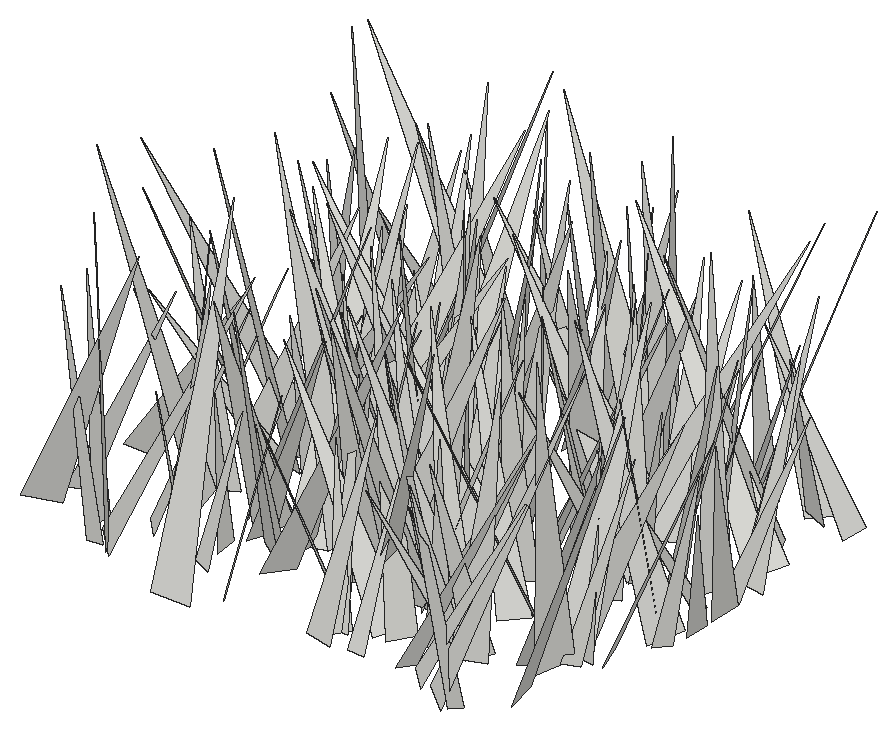
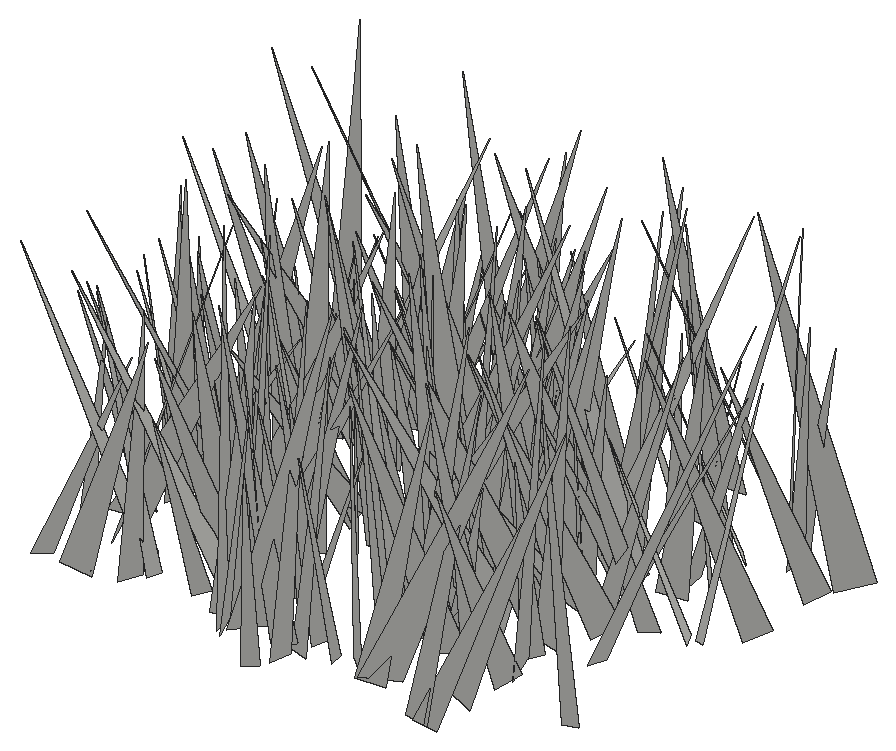
# SketchUp Ruby script. Lengths in inches.
U = 1.inch
M = Sketchup.active_model
def pt(a) = Geom::Point3d.new(a.map { |v| v * U })
def face(e, loops, mat)
  f = e.add_face(loops[0].map { |a| pt(a) })
  loops[1..].each { |l| e.add_face(l.map { |a| pt(a) }).erase! }
  f.material = f.back_material = mat if mat
  f
end
# faces: each face lists its corners as indices into pts; further lists are holes
def faces(e, pts, list, mat = nil) = list.each { |f| face(e, (f[0].is_a?(Array) ? f : [f]).map { |l| l.map { |i| pts[i] } }, mat) }
# xy, xz, yz: faces in a plane at the given z, y or x. An outline is a flat list of corners, or four numbers for a rectangle; further outlines are holes
def ring(l) = l.size == 4 ? [[l[0], l[1]], [l[2], l[1]], [l[2], l[3]], [l[0], l[3]]] : l.each_slice(2).to_a
def flat(e, list, mat, &to3) = list.each { |f| face(e, (f[0].is_a?(Array) ? f : [f]).map { |l| ring(l).map { |u, v| to3.(u, v) } }, mat) }
def xy(e, z, list, mat = nil) = flat(e, list, mat) { |x, y| [x, y, z] }
def xz(e, y, list, mat = nil) = flat(e, list, mat) { |x, z| [x, y, z] }
def yz(e, x, list, mat = nil) = flat(e, list, mat) { |y, z| [x, y, z] }
def lines(e, pts, list) = list.each { |a, b| e.add_line(pt(pts[a]), pt(pts[b])) }
# prism: a flat outline (further loops are holes) pulled along v
def prism(e, loops, v, mat = nil)
  f = face(e, loops, mat); d = Geom::Vector3d.new(v.map { |x| x * U })
  f.pushpull(f.normal.samedirection?(d) ? d.length : -d.length)
end
def box(e, o, s, mat = nil) = prism(e, [[o, [o[0] + s[0], o[1], o[2]], [o[0] + s[0], o[1] + s[1], o[2]], [o[0], o[1] + s[1], o[2]]]], [0, 0, s[2]], mat)
def at(x, y, z, deg = 0) = Geom::Transformation.translation(pt([x, y, z])) * Geom::Transformation.rotation(ORIGIN, Z_AXIS, deg.degrees)
def axes(o, x, y, z) = Geom::Transformation.new([*x, 0, *y, 0, *z, 0, *pt(o).to_a, 1])
def part(name) = M.definitions.add(name)
# library, detail: a bought-in or finely detailed component or shape, given as its bounding box
def library(name, o, s) = part(name).tap { |d| box(d.entities, o, s) }
def detail(e, o, s) = box(e.add_group.entities, o, s)
def put(e, d, t, mat = nil) = e.add_instance(d, t).tap { |i| i.material = mat if mat }
def group(e, t, mat = nil) = e.add_group.tap { |g| g.transformation = t; g.material = mat if mat }.entities
root = M.entities
c1 = part("fur_instance\#9")
p = [[0.8125,0,1.79],[0.67,-0.02,1.48],[0,-0.11,0],[0,0.11,0]]
faces(c1.entities,p,[[0,1,2,3]])
put(root,c1,axes([148.23,376.57,-27.1],[0.29151,4.89673,1.62599],[5.06271,0.04273,-1.03633],[0.99541,-1.65136,4.79468]))
put(root,c1,axes([153.89,377.34,-27.1],[-3.07283,-1.79032,0.75021],[-1.87261,3.10397,-0.26279],[0.51124,0.60869,3.54662]))
put(root,c1,axes([153.01,376.6,-27.1],[3.55975,3.91646,0.08522],[3.79537,-3.41954,-1.38552],[0.97011,-0.99289,5.10792]))
put(root,c1,axes([141.76,376.98,-27.1],[-3.37291,-1.64413,0.77782],[-1.79286,3.28135,-0.83849],[0.30629,1.10194,3.65741]))
put(root,c1,axes([141.93,375.51,-27.1],[-0.24232,8.0833,1.63068],[8.24361,0.27788,-0.15248],[0.20433,-1.625,8.08549]))
put(root,c1,axes([137.36,377.47,-27.1],[-5.46878,-3.64969,2.6695],[-4.02035,5.84198,-0.2491],[2.0696,1.70441,6.57007]))
put(root,c1,axes([154.51,375.8,-27.1],[4.64022,6.0526,0.40907],[6.0581,-4.59639,-0.71102],[0.31728,-0.75645,7.59342]))
put(root,c1,axes([133.34,378.5,-27.1],[5.01421,-5.55154,0.43768],[-5.45899,-4.78379,1.86233],[1.10028,1.565,7.24525]))
put(root,c1,axes([137.01,377.11,-27.1],[-2.00481,-4.221,2.16779],[-4.72189,1.54205,-1.3643],[-0.46899,2.51807,4.46932]))
put(root,c1,axes([155.55,375.68,-27.1],[-6.80362,-1.51626,0.05987],[-1.39466,6.13985,-2.9915],[-0.59797,2.93174,6.29597]))
put(root,c1,axes([148.56,377.52,-27.1],[-3.29969,1.99263,1.18367],[2.06312,3.46364,-0.07948],[1.05601,-0.54058,3.85386]))
put(root,c1,axes([152.93,379.34,-27.1],[-3.89152,-1.38284,0.09587],[-1.31779,3.77936,1.02238],[0.42995,-0.93252,4.00136]))
put(root,c1,axes([153.84,379.32,-27.1],[3.33283,-3.55166,1.19436],[-3.37517,-3.53973,-1.10774],[-1.62758,0.06765,4.74288]))
put(root,c1,axes([143.4,376.95,-27.1],[3.40494,2.47984,0.75094],[2.39973,-3.48584,0.63038],[-0.97714,0.08048,4.16483]))
put(root,c1,axes([152.64,379.25,-27.1],[-3.58815,0.95471,1.93369],[1.59157,3.70529,1.12394],[1.45517,-1.69849,3.5388]))
put(root,c1,axes([148.56,379.69,-27.1],[7.85727,-0.11013,0.63762],[0.0287,-7.70188,-1.68396],[-0.64642,-1.6806,7.67549]))
put(root,c1,axes([156.96,377.9,-27.1],[7.02887,1.41814,0.69885],[1.44367,-7.05544,-0.2028],[-0.64447,-0.3379,7.16763]))
put(root,c1,axes([149.99,376.61,-27.1],[0.7,4.04155,0.09862],[4.02713,-0.70587,0.34334],[-0.35517,-0.03822,4.08733]))
put(root,c1,axes([137.3,377.45,-27.1],[4.92095,5.18553,0.33695],[5.09859,-4.72846,-1.69263],[1.00379,-1.4039,6.94554]))
put(root,c1,axes([152.1,377.04,-27.1],[5.39304,-0.33096,0.39775],[-0.43435,-5.15892,1.59671],[-0.28121,1.6213,5.16187]))
put(root,c1,axes([148,378.51,-27.1],[-3.22375,-2.36609,0.00506],[-2.25529,3.0702,-1.21594],[-0.71558,0.9831,3.80952]))
put(root,c1,axes([152.02,379.0625,-27.1],[3.93082,-2.70083,1.38603],[-2.7651,-4.12134,-0.18897],[-1.2529,0.6221,4.76552]))
put(root,c1,axes([139.46,378.93,-27.1],[-0.7765,-5.95979,2.50914],[-6.25232,1.3369,1.24057],[1.65027,2.26084,5.88073]))
put(root,c1,axes([136.2,378.5,-27.1],[-5.05567,-0.39861,1.84756],[-0.46846,5.37567,-0.1221],[1.83109,0.27472,5.06989]))
put(root,c1,axes([148.35,377.54,-27.1],[0.28645,5.00767,1.03913],[5.08565,-0.389,0.47271],[-0.54104,-1.00525,4.99354]))
put(root,c1,axes([141.27,378.24,-27.1],[1.148,3.43718,0.90942],[3.54891,-1.0498,-0.51218],[0.21566,-1.0212,3.58745]))
put(root,c1,axes([149.99,378.6875,-27.1],[-4.53112,4.00144,0.54603],[3.94801,4.21612,1.86503],[-0.85024,-1.74745,5.75015]))
put(root,c1,axes([153.67,378.85,-27.1],[3.4619,-5.09824,2.22403],[-5.52391,-3.4582,0.67108],[-0.65172,2.22978,6.12588]))
put(root,c1,axes([156.52,380.46,-27.1],[6.94101,-3.43299,1.84422],[-3.2352,-7.17632,-1.18245],[-2.17258,-0.28153,7.65277]))
put(root,c1,axes([142.72,380.66,-27.1],[-2.91514,-5.53327,1.42514],[-5.42873,3.18122,1.24695],[1.78243,0.63944,6.12864]))
put(root,c1,axes([141.09,379.92,-27.1],[3.87563,-0.57439,1.14349],[-0.32332,-3.96837,-0.89752],[-1.23813,-0.76168,3.81378]))
put(root,c1,axes([147.22,381.04,-27.1],[1.68994,-6.65431,0.98946],[-6.7239,-1.70391,0.02495],[-0.21912,0.96522,6.8655]))
put(root,c1,axes([149.86,380.96,-27.1],[-1.24664,-7.42641,1.30497],[-7.49381,1.07378,-1.04811],[-0.83512,1.45053,7.45702]))
put(root,c1,axes([141.66,382.16,-27.1],[5.49992,-4.64771,0.52674],[-4.40214,-5.41809,-1.84207],[-1.58109,-1.08206,6.96111]))
put(root,c1,axes([152.46,380.15,-27.1],[-7.15146,0.58689,0.88826],[0.71619,7.11549,1.06478],[0.78773,-1.14116,7.09606]))
put(root,c1,axes([155.46,381.56,-27.1],[-4.1792,-5.61615,0.15739],[-5.61189,4.16336,-0.45249],[-0.26934,0.3962,6.98585]))
put(root,c1,axes([143.77,379.72,-27.1],[7.07032,-2.50038,0.22823],[-2.5064,-6.98854,1.08245],[0.14815,1.09629,7.42089]))
put(root,c1,axes([143.08,380.72,-27.1],[-3.69542,-5.95234,1.80806],[-6.20183,3.68953,-0.52934],[0.48649,1.82006,6.98615]))
put(root,c1,axes([146.64,380.12,-27.1],[-2.09497,-3.98677,2.51489],[-4.46346,2.56262,0.34425],[1.51546,2.03632,4.49052]))
put(root,c1,axes([137.96,379.41,-27.1],[3.6626,3.70148,0.35684],[3.71844,-3.64024,-0.40601],[0.03906,-0.53912,5.19141]))
put(root,c1,axes([150.67,378.57,-27.1],[-7.44461,1.33123,0.56849],[1.18187,7.30967,-1.63995],[0.83578,1.52121,7.38274]))
put(root,c1,axes([141.6,381.41,-27.1],[5.62437,-1.82953,0.08499],[-1.8284,-5.62476,-0.0835],[-0.10665,-0.05312,5.91386]))
put(root,c1,axes([133.94,380.01,-27.1],[4.38543,-2.43855,0.87514],[-2.59033,-4.09309,1.5752],[0.05089,1.80126,4.76417]))
put(root,c1,axes([142.1,382.875,-27.1],[-4.63636,-6.55031,0.51962],[-6.56307,4.58532,-0.75728],[-0.32055,0.86066,7.9893]))
put(root,c1,axes([138.32,382.1875,-27.1],[-7.66466,-1.90179,1.421],[-1.79066,7.78455,0.75987],[1.55871,-0.40873,7.86043]))
put(root,c1,axes([147.3125,382.53,-27.1],[-0.33805,-5.61743,0.95415],[-5.65981,0.22074,-0.70569],[-0.6576,0.9879,5.58317]))
put(root,c1,axes([146.99,381.77,-27.1],[-2.52237,2.99386,0.77548],[2.99232,2.10973,1.58806],[-0.78138,-1.58517,3.57821]))
put(root,c1,axes([151.04,381.375,-27.1],[3.04965,-4.5466,3.26672],[-5.09549,-3.79519,-0.52522],[-2.31926,2.35973,5.44941]))
put(root,c1,axes([150.29,381.64,-27.1],[4.26333,-3.02404,0.31767],[-2.97687,-4.03955,1.49732],[0.61963,1.39963,5.00788]))
put(root,c1,axes([137.4,382.14,-27.1],[4.80931,3.10321,2.02961],[3.46778,-4.94111,-0.66234],[-1.31293,-1.68352,5.68513]))
put(root,c1,axes([147.29,383.14,-27.1],[-7.26006,2.55391,1.83228],[2.95803,7.11093,1.80912],[1.0629,-2.34529,7.48051]))
put(root,c1,axes([149.7,383.16,-27.1],[-4.06839,-1.50308,0.30492],[-1.46625,4.06536,0.47647],[0.44983,-0.34301,4.31092]))
put(root,c1,axes([149.56,381.15,-27.1],[4.3993,3.63087,0.47155],[3.65139,-4.40515,-0.14642],[-0.27004,-0.41338,5.70225]))
put(root,c1,axes([143.54,381.74,-27.1],[4.7353,0.6555,1.15241],[0.55235,-4.8611,0.49538],[-1.20525,0.34759,4.75472]))
put(root,c1,axes([157.65,382.35,-27.1],[5.84375,1.80801,0.13219],[1.81029,-5.79638,-0.74876],[0.09603,-0.75425,6.07105]))
put(root,c1,axes([140.02,383.17,-27.1],[8.09633,1.85359,0.38508],[1.89305,-7.94545,-1.5559],[-0.02113,-1.6027,8.15877]))
put(root,c1,axes([146.75,382.48,-27.1],[1.17731,-6.81979,2.88625],[-6.91612,0.0321,2.89694],[2.64712,3.11697,6.28517]))
put(root,c1,axes([156.87,380.98,-27.1],[3.7026,-0.58317,1.91769],[-1.4169,-3.61072,1.63767],[-1.41775,2.08554,3.37155]))
put(root,c1,axes([144.97,383.7,-27.1],[-5.38028,-3.08502,1.66928],[-3.07413,5.61908,0.47644],[1.68926,0.39986,6.18367]))
put(root,c1,axes([157.23,381.55,-27.1],[1.77865,4.09096,1.0407],[3.89915,-2.02489,1.29578],[-1.61729,-0.38272,4.26855]))
put(root,c1,axes([146.23,381.42,-27.1],[3.62964,3.56201,0.97293],[3.43547,-3.75775,0.94107],[-1.35352,0.01415,4.99765]))
put(root,c1,axes([138.33,383.3,-27.1],[1.39978,-5.30319,2.32473],[-5.64349,-1.78474,-0.67328],[-1.29585,2.04412,5.44334]))
put(root,c1,axes([153.04,382.375,-27.1],[-3.19469,4.99874,1.10839],[5.10889,3.02549,1.08057],[-0.33936,-1.5103,5.83317]))
put(root,c1,axes([155.4,383.52,-27.1],[1.83372,-5.8574,1.52699],[-5.60076,-1.03656,2.74963],[2.29617,2.14936,5.48737]))
put(root,c1,axes([135.29,385.45,-27.1],[-2.98193,-4.15353,0.46379],[-3.81224,2.9367,1.78925],[1.71281,-0.69483,4.78981]))
put(root,c1,axes([144.36,386.08,-27.1],[-0.43827,-6.52973,0.002],[-6.42899,0.43186,1.145],[1.14256,-0.07472,6.44348]))
put(root,c1,axes([133.84,383.74,-27.1],[3.57334,-4.4658,0.19156],[-4.12422,-3.19939,2.34597],[1.72363,1.60293,5.21618]))
put(root,c1,axes([146.41,381.99,-27.1],[-6.04879,4.39479,0.23194],[4.40071,6.03643,0.38865],[-0.04117,-0.45072,7.46666]))
put(root,c1,axes([144.76,384.87,-27.1],[1.52104,-3.59534,0.18519],[-3.58042,-1.53172,-0.32978],[-0.37596,0.04131,3.88989]))
put(root,c1,axes([144.45,383.03,-27.1],[-8.05212,1.79962,1.36323],[1.82873,8.16018,0.02927],[1.32393,-0.32629,8.25072]))
put(root,c1,axes([156.2,381.98,-27.1],[-1.91497,6.86191,1.78883],[6.91485,2.21764,-1.10438],[1.57179,-1.39609,7.03799]))
put(root,c1,axes([146.48,381.42,-27.1],[-5.7713,0.32455,0.04644],[0.28097,5.31808,-2.2482],[0.16895,2.24233,5.3253]))
put(root,c1,axes([155.48,379.83,-27.1],[6.83312,3.40706,1.30672],[2.45514,-6.34476,3.70451],[-2.69961,2.8536,6.67654]))
put(root,c1,axes([138.86,386.01,-27.1],[-4.92347,-1.39259,0.14711],[-1.23579,4.5738,1.93769],[0.65861,-1.82825,4.73553]))
put(root,c1,axes([147.97,383.09,-27.1],[-5.43325,1.77797,0.85582],[1.73658,5.49897,-0.39929],[0.93695,0.1182,5.7028]))
put(root,c1,axes([158.37,384.84,-27.1],[-6.07802,2.92755,1.98205],[3.37511,5.97833,1.51972],[1.05246,-2.26504,6.57292]))
put(root,c1,axes([151.33,384.84,-27.1],[-3.30956,4.62511,3.28339],[5.43338,3.67626,0.29816],[1.62808,-2.86687,5.67942]))
put(root,c1,axes([146.87,385.1,-27.1],[-1.94061,6.26278,4.61542],[7.19839,3.24975,-1.38302],[2.95087,-3.80883,6.40903]))
put(root,c1,axes([144.56,384.34,-27.1],[0.81184,5.62301,2.88886],[5.96448,-1.64652,1.52868],[-2.09495,-2.50871,5.47179]))
put(root,c1,axes([158.71,384.22,-27.1],[3.49135,-1.63355,1.08284],[-1.80913,-3.53699,0.49727],[-0.7537,0.9229,3.8224]))
put(root,c1,axes([159,385.9375,-27.1],[3.9114,-1.46291,0.01114],[-1.40736,-3.77134,-1.11157],[-0.39945,-1.03737,4.02536]))
put(root,c1,axes([140.84,385.68,-27.1],[2.96444,-3.24193,0.90441],[-3.19075,-3.09049,-0.61962],[-1.07107,0.23387,4.34903]))
put(root,c1,axes([148.3125,386.05,-27.1],[-7.32197,2.2534,1.35544],[2.57225,6.97064,2.30649],[0.54639,-2.61889,7.30542]))
put(root,c1,axes([154.31,387.31,-27.1],[-5.03232,-2.4099,0.87584],[-1.92345,4.82363,2.22078],[1.6956,-1.68045,5.11859]))
put(root,c1,axes([156.44,386.59,-27.1],[-3.5454,-4.09399,1.47684],[-3.82101,3.83994,1.47185],[2.08366,0.07566,5.21193]))
put(root,c1,axes([145.8125,386.08,-27.1],[3.71105,4.69804,3.51461],[5.68502,-3.90755,-0.77947],[-1.45074,-3.29476,5.93598]))
put(root,c1,axes([139.26,384.36,-27.1],[4.45979,0.0367,0.09292],[0.01604,-4.35825,0.95137],[-0.0986,0.95079,4.35729]))
put(root,c1,axes([141.31,385.03,-27.1],[2.46567,3.17158,1.58955],[3.37143,-2.69731,0.15219],[-1.10413,-1.15357,4.01439]))
put(root,c1,axes([154.62,385.73,-27.1],[3.53738,-5.32848,1.99163],[-5.66565,-3.51029,0.67133],[-0.50966,2.039,6.36044]))
put(root,c1,axes([150.43,385.19,-27.1],[6.68807,0.43229,0.66728],[0.41432,-6.71942,0.20043],[-0.67859,0.15798,6.69903]))
put(root,c1,axes([143.47,381.84,-27.1],[-6.01479,5.28528,0.0687],[5.03484,5.76049,-2.36301],[1.60915,1.73181,7.65037]))
put(root,c1,axes([143.72,388.47,-27.1],[5.51839,-2.97407,0.09463],[-2.75984,-5.19025,-2.17974],[-1.11235,-1.87694,5.87762]))
put(root,c1,axes([143.98,385.17,-27.1],[0.77097,6.55392,2.92574],[6.60675,-1.79779,2.28627],[-2.8044,-2.43357,6.19042]))
put(root,c1,axes([158.96,387.67,-27.1],[5.13341,-1.95182,0.40555],[-1.78394,-4.9977,-1.47188],[-0.88973,-1.24068,5.29103]))
put(root,c1,axes([146.28,385.23,-27.1],[4.52049,-0.19473,1.20973],[-0.39564,-4.60837,0.73662],[-1.15967,0.81315,4.46432]))
put(root,c1,axes([145.81,384.18,-27.1],[-1.08496,4.24211,0.2137],[4.12597,1.10497,-0.98676],[1.00871,0.04308,4.26602]))
put(root,c1,axes([135.72,385.55,-27.1],[3.83341,2.26597,0.28943],[2.28132,-3.82668,-0.25597],[-0.11822,-0.36786,4.44568]))
put(root,c1,axes([139.32,386.2,-27.1],[-3.64938,-5.29226,1.74557],[-5.55344,3.28039,-1.66476],[-0.463,2.36729,6.20923]))
put(root,c1,axes([144.82,386.66,-27.1],[5.44749,2.02001,0.26599],[2.02291,-5.27178,-1.39377],[0.24298,-1.39796,5.64031]))
put(root,c1,axes([150.3,385.48,-27.1],[0.9151,5.15761,1.58711],[5.35443,-1.06795,0.38322],[-0.67079,-1.48856,5.22413]))
put(root,c1,axes([152.88,387.36,-27.1],[3.69815,0.46024,1.83595],[1.02421,-3.87534,-1.09159],[-1.5917,-1.42435,3.56322]))
put(root,c1,axes([137.25,386,-27.1],[1.94999,6.06367,1.85826],[6.06829,-1.21894,-2.39034],[1.84311,-2.40204,5.90397]))
put(root,c1,axes([137.34,389.04,-27.1],[-7.29024,-1.74958,0.87658],[-1.40156,7.02793,2.37084],[1.36568,-2.12702,7.11251]))
put(root,c1,axes([142.7,385.83,-27.1],[-2.8521,5.31504,2.52319],[5.50682,3.39878,-0.93481],[2.07151,-1.71732,5.95905]))
put(root,c1,axes([158,387.35,-27.1],[-0.53868,-3.7535,0.51973],[-3.36849,0.23389,-1.80211],[-1.73555,0.71104,3.33637]))
put(root,c1,axes([151.36,385.9375,-27.1],[3.9948,0.59542,0.26899],[0.55235,-3.96784,0.58004],[-0.34899,0.53573,3.99706]))
put(root,c1,axes([152.68,387.78,-27.1],[-4.88015,-2.78524,1.52655],[-2.68194,5.11285,0.7548],[1.7015,0.07051,5.5681]))
put(root,c1,axes([154.36,385.53,-27.1],[4.62309,3.63215,1.82021],[3.50208,-4.96051,1.00367],[-2.05939,-0.28182,5.79293]))
put(root,c1,axes([147.66,386.93,-27.1],[-6.42815,4.45601,0.04956],[4.21627,6.0534,2.59983],[-1.44275,-2.16333,7.37686]))
put(root,c1,axes([151.31,389.31,-27.1],[4.3126,-6.65441,0.44802],[-6.65528,-4.32849,-0.22777],[-0.435,0.25174,7.9264]))
put(root,c1,axes([147.5625,386.39,-27.1],[-5.47988,-2.79163,2.54101],[-3.31815,5.69792,-0.89593],[1.79996,2.00489,6.08438]))
put(root,c1,axes([154.83,387.72,-27.1],[4.24921,-1.39082,0.67887],[-1.35455,-4.30166,-0.33452],[-0.74864,-0.11098,4.4585]))
put(root,c1,axes([156.4375,387.76,-27.1],[5.73568,-0.06882,1.05766],[0.01363,-5.81521,-0.45231],[-1.05981,-0.44725,5.71823]))
put(root,c1,axes([138.55,386.99,-27.1],[4.87522,-3.55324,0.35007],[-3.38958,-4.41978,2.34354],[1.12198,2.08707,5.55888]))
put(root,c1,axes([154.69,388.2,-27.1],[-6.88709,2.46248,0.81316],[2.58785,6.67518,1.70354],[0.16756,-1.88022,7.11293]))
put(root,c1,axes([141.51,385.69,-27.1],[3.64416,1.65962,0.06909],[1.4569,-3.27351,1.789],[-0.79783,1.60274,3.58241]))
put(root,c1,axes([149.46,388.39,-27.1],[4.52719,2.71843,2.25301],[3.1828,-4.72799,-0.69084],[-1.52829,-1.79378,5.23527]))
put(root,c1,axes([156.55,387.34,-27.1],[4.95919,2.18923,1.00137],[2.21006,-5.04934,0.09393],[-0.95452,-0.31696,5.4201]))
put(root,c1,axes([149.01,387.45,-27.1],[1.36969,7.27883,2.41401],[7.66649,-1.2409,-0.6083],[0.18385,-2.48268,7.38156]))
put(root,c1,axes([143.18,388.48,-27.1],[4.24569,0.44069,0.96407],[0.53821,-4.32495,-0.39327],[-0.91322,-0.50013,4.25034]))
put(root,c1,axes([146.86,387.35,-27.1],[3.58302,-2.92408,2.58959],[-3.63927,-3.77537,0.77237],[-1.41842,2.30013,4.5598]))
put(root,c1,axes([139.69,389.17,-27.1],[1.75829,5.41715,3.42251],[6.36736,-1.87488,-0.30363],[-0.71818,-3.36006,5.68726]))
put(root,c1,axes([141.34,387.59,-27.1],[2.97178,5.39968,0.42783],[5.06638,-2.59832,-2.39825],[1.91609,-1.5044,5.67771]))
put(root,c1,axes([146.77,388.42,-27.1],[4.56446,-0.76979,0.5853],[-0.81155,-4.58493,0.29877],[-0.52586,0.39409,4.61927]))
put(root,c1,axes([146,389.68,-27.1],[4.04324,-6.81137,0.9787],[-6.74817,-3.70246,2.11055],[1.34718,1.89668,7.63467]))
put(root,c1,axes([151.41,385.875,-27.1],[5.35308,0.77922,1.1136],[0.09871,-4.73607,2.83947],[-1.35556,2.73224,4.60435]))
put(root,c1,axes([141.13,386.19,-27.1],[1.53253,6.73152,0.42824],[6.72346,-1.5597,0.45586],[-0.5402,-0.31526,6.8887]))
put(root,c1,axes([143.18,390.76,-27.1],[7.23074,-0.77372,0.74856],[-0.57311,-7.06946,-1.77111],[-0.91134,-1.69312,7.05304]))
put(root,c1,axes([157.55,388.8125,-27.1],[6.19428,-1.57461,3.33029],[-1.87234,-6.95675,0.19327],[-3.17247,1.03131,6.38836]))
put(root,c1,axes([158.33,388.92,-27.1],[1.81296,4.05322,0.9149],[4.0683,-1.5284,-1.29051],[0.84535,-1.3371,4.24853]))
put(root,c1,axes([156.49,388.8125,-27.1],[4.35259,2.65064,0.87547],[2.69973,-4.40951,-0.0717],[-0.70982,-0.51745,5.09567]))
put(root,c1,axes([151.92,390.47,-27.1],[-3.79405,-1.81524,0.00607],[-1.81515,3.79397,0.03081],[0.01877,-0.02517,4.20582]))
put(root,c1,axes([153.38,389.28,-27.1],[-1.15441,5.11883,1.74969],[5.40957,1.09949,0.35248],[0.0216,-1.78472,5.23554]))
put(root,c1,axes([141.09,387.87,-27.1],[-0.22471,7.89617,1.63504],[7.5306,0.79034,-2.78188],[2.88322,-1.44886,7.39332]))
put(root,c1,axes([143.38,390.35,-27.1],[1.79677,-5.19077,1.98742],[-5.55817,-1.66844,0.66734],[0.02536,2.09632,5.45226]))
put(root,c1,axes([144.99,388.58,-27.1],[-0.16365,8.04006,1.71484],[8.20749,0.06185,0.49328],[-0.46944,-1.72152,8.02659]))
put(root,c1,axes([151.82,389.43,-27.1],[1.21689,3.56799,0.58582],[3.55761,-1.29191,0.47847],[-0.64586,-0.39367,3.73931]))
put(root,c1,axes([143.25,390,-27.1],[-2.90723,2.3787,0.42473],[2.40963,2.90345,0.23285],[0.1797,-0.4498,3.74913]))
put(root,c1,axes([158.53,389.8,-27.1],[0.17579,4.7582,1.26729],[4.89735,-0.03702,-0.54033],[0.51227,-1.27889,4.73069]))
put(root,c1,axes([139.47,390.26,-27.1],[-3.40994,2.09099,1.78678],[2.1335,3.80705,-0.3836],[1.73581,-0.57158,3.98156]))
put(root,c1,axes([152.39,390.94,-27.1],[-4.17203,-5.0841,2.64194],[-5.48144,4.49304,-0.00972],[1.66784,2.04897,6.57676]))
put(root,c1,axes([143.81,392.625,-27.1],[7.53646,1.85279,1.2332],[2.16443,-7.11553,-2.53698],[-0.51849,-2.77277,7.33449]))
put(root,c1,axes([156.35,390.42,-27.1],[3.88828,4.27161,1.82836],[4.44707,-4.1121,0.14976],[-1.3465,-1.2459,5.77433]))
put(root,c1,axes([151.5,392.2,-27.1],[-6.98354,0.71492,0.27676],[0.75932,6.7998,1.59491],[0.10557,-1.6153,6.83646]))
put(root,c1,axes([157.6,392.7,-27.1],[-6.20771,-3.16783,0.82777],[-3.08728,6.25411,0.78157],[1.09042,-0.32718,6.92531]))
put(root,c1,axes([149.4,392.4375,-27.1],[-6.05597,0.77226,2.0179],[1.21073,6.18666,1.26588],[1.78953,-1.57224,5.97233]))
put(root,c1,axes([152.47,389.86,-27.1],[3.82071,6.83533,0.31448],[6.59967,-3.58608,-2.23672],[1.80694,-1.35528,7.50444]))
put(root,c1,axes([143.7,391.81,-27.1],[-6.59669,1.20746,2.1658],[1.44471,6.87425,0.5679],[2.0153,-0.97558,6.6822]))
put(root,c1,axes([142.8,389.66,-27.1],[-0.26987,6.47949,0.83868],[6.52839,0.23411,0.29205],[-0.25936,-0.84936,6.47853]))
put(root,c1,axes([139.26,391.24,-27.1],[-7.32615,-2.19993,2.60741],[-2.57876,7.61493,-0.82074],[2.23345,1.57604,7.60517]))
put(root,c1,axes([158.22,391.1875,-27.1],[-5.28258,5.45364,0.12335],[5.18528,4.96674,2.47132],[-1.69419,-1.80343,7.17917]))
put(root,c1,axes([153.84,390.68,-27.1],[3.74309,-3.05687,3.19875],[-4.02453,-4.09315,0.7978],[-1.83838,2.73658,4.76642]))
put(root,c1,axes([158.2,390.1,-27.1],[1.54833,5.59255,0.52827],[5.59137,-1.58705,0.41342],[-0.54067,-0.39706,5.78818]))
put(root,c1,axes([150.07,393.07,-27.1],[2.36521,-5.47601,0.71506],[-5.30162,-2.03369,1.96193],[1.54624,1.40343,5.6331]))
put(root,c1,axes([135.09,393.49,-27.1],[-1.49518,-5.85947,1.8909],[-5.5495,2.12534,2.19783],[2.66683,1.13753,5.63369]))
put(root,c1,axes([141.99,388.63,-27.1],[7.42778,3.7642,0.92799],[3.25227,-7.14156,2.93652],[-2.11023,2.24305,7.79217]))
put(root,c1,axes([148.11,392.96,-27.1],[-3.79704,-0.30553,0.54536],[-0.26679,3.82814,0.28712],[0.56533,-0.2455,3.79848]))
put(root,c1,axes([141.41,391.4,-27.1],[-2.96108,3.10315,0.36366],[3.04624,2.97875,-0.6142],[0.69442,0.16515,4.24503]))
put(root,c1,axes([148.73,392.08,-27.1],[-3.00951,3.51493,1.30262],[3.55292,3.20728,-0.44587],[1.1951,-0.68362,4.60577]))
put(root,c1,axes([153.36,391.19,-27.1],[-2.46279,4.53865,0.90199],[4.34757,2.61941,-1.3098],[1.58479,-0.13272,4.99491]))
put(root,c1,axes([154.54,394.22,-27.1],[5.4983,0.81734,0.21266],[0.84397,-5.26527,-1.58403],[0.03145,-1.59793,5.32824]))
put(root,c1,axes([144.1,393.49,-27.1],[5.56182,2.46032,2.03104],[2.73268,-5.78042,-0.48104],[-1.64644,-1.28288,6.06264]))
put(root,c1,axes([139.67,394.54,-27.1],[-1.62801,-6.13851,1.48062],[-6.15059,1.19536,-1.80699],[-1.42958,1.84764,6.08822]))
put(root,c1,axes([146.36,394.27,-27.1],[5.46664,-0.56538,0.68203],[-0.51758,-5.49848,-0.40957],[-0.71898,-0.34055,5.48051]))
put(root,c1,axes([157.04,395.49,-27.1],[-0.66532,-4.77379,0.4836],[-4.67341,0.75535,1.0268],[1.0873,0.32553,4.70929]))
put(root,c1,axes([153.01,392.16,-27.1],[6.48449,2.8801,0.19854],[2.8437,-6.45643,0.78158],[-0.49773,0.63448,7.05214]))
put(root,c1,axes([142.17,391.95,-27.1],[-2.25135,6.36064,1.32657],[6.19225,2.52565,-1.60099],[1.96812,-0.67041,6.55463]))
put(root,c1,axes([138.99,392.34,-27.1],[-4.17558,2.72173,1.55923],[2.19552,4.39009,-1.78362],[2.24025,0.77057,4.65424]))
put(root,c1,axes([146.53,395.53,-27.1],[-2.50316,-5.2047,1.47138],[-5.2002,2.76171,0.92225],[1.48721,0.89649,5.70124]))
put(root,c1,axes([143.03,395.58,-27.1],[1.51569,-5.39227,1.25729],[-5.41404,-1.71643,-0.83467],[-1.15995,0.96539,5.5387]))
put(root,c1,axes([155.1,394.98,-27.1],[-4.81176,0.83188,2.6308],[1.27412,5.3609,0.63523],[2.44739,-1.15538,4.84165]))
put(root,c1,axes([152.3,394.17,-27.1],[2.6099,-2.39325,0.8726],[-2.54736,-2.4537,0.88934],[-0.00348,1.24593,3.42758]))
put(root,c1,axes([150.16,395.43,-27.1],[7.38345,1.68053,2.79244],[2.22073,-7.65548,-1.26461],[-2.38543,-1.92527,7.46594]))
put(root,c1,axes([149.39,393.75,-27.1],[-4.16278,-2.64249,2.71758],[-3.23685,4.57857,-0.50613],[1.97251,1.93665,4.90462]))
put(root,c1,axes([150.39,395.02,-27.1],[1.19646,-6.35488,2.45253],[-6.76034,-1.41301,-0.36331],[-0.83491,2.33448,6.45631]))
put(root,c1,axes([142.91,395.16,-27.1],[-7.09229,4.18803,1.11711],[4.32642,6.70959,2.31334],[-0.26383,-2.55536,7.90497]))
put(root,c1,axes([158.95,395.49,-27.1],[-4.51725,1.3418,0.80765],[1.52463,4.33149,1.33117],[0.35811,-1.51528,4.52039]))
put(root,c1,axes([146.88,396.21,-27.1],[6.67439,0.3641,2.55328],[0.99441,-6.8993,-1.61558],[-2.3797,-1.86182,6.48614]))
put(root,c1,axes([147.42,395.29,-27.1],[0.1838,-6.38239,2.38865],[-6.46729,0.58989,2.0738],[2.14821,2.32195,6.03888]))
put(root,c1,axes([139.86,396.79,-27.1],[-1.86711,-6.21996,0.83765],[-6.21183,1.95621,0.67975],[0.89595,0.60083,6.45848]))
put(root,c1,axes([145.15,395.03,-27.1],[3.94564,1.0984,0.79467],[1.2,-3.96752,-0.47419],[-0.63087,-0.67703,4.06813]))
put(root,c1,axes([155.21,393.54,-27.1],[6.72288,3.05704,0.61475],[3.02645,-6.7488,0.46346],[-0.75102,0.16938,7.37074]))
put(root,c1,axes([149.29,395.19,-27.1],[-7.00283,2.97011,1.6591],[3.21934,7.01289,1.03394],[1.10002,-1.61605,7.53606]))
put(root,c1,axes([139.37,396.9,-27.1],[1.40326,-4.201,0.43994],[-3.89786,-1.46649,-1.57071],[-1.62745,-0.10993,4.1413]))
put(root,c1,axes([144.1875,394.94,-27.1],[3.38997,4.6985,2.258],[4.82742,-3.84601,0.75539],[-1.96736,-1.34115,5.74432]))
put(root,c1,axes([150,395.65,-27.1],[-4.89428,-1.48699,1.50253],[-1.73277,4.99254,-0.70337],[1.21087,1.13406,5.0666]))
put(root,c1,axes([157.14,395.71,-27.1],[-2.40654,5.51072,1.54274],[5.60544,1.9331,1.83892],[-1.15197,-2.10585,5.72519]))
put(root,c1,axes([147.37,397.41,-27.1],[0.94706,-3.59902,0.23008],[-3.53322,-0.8783,0.80484],[0.72266,0.42244,3.63347]))
